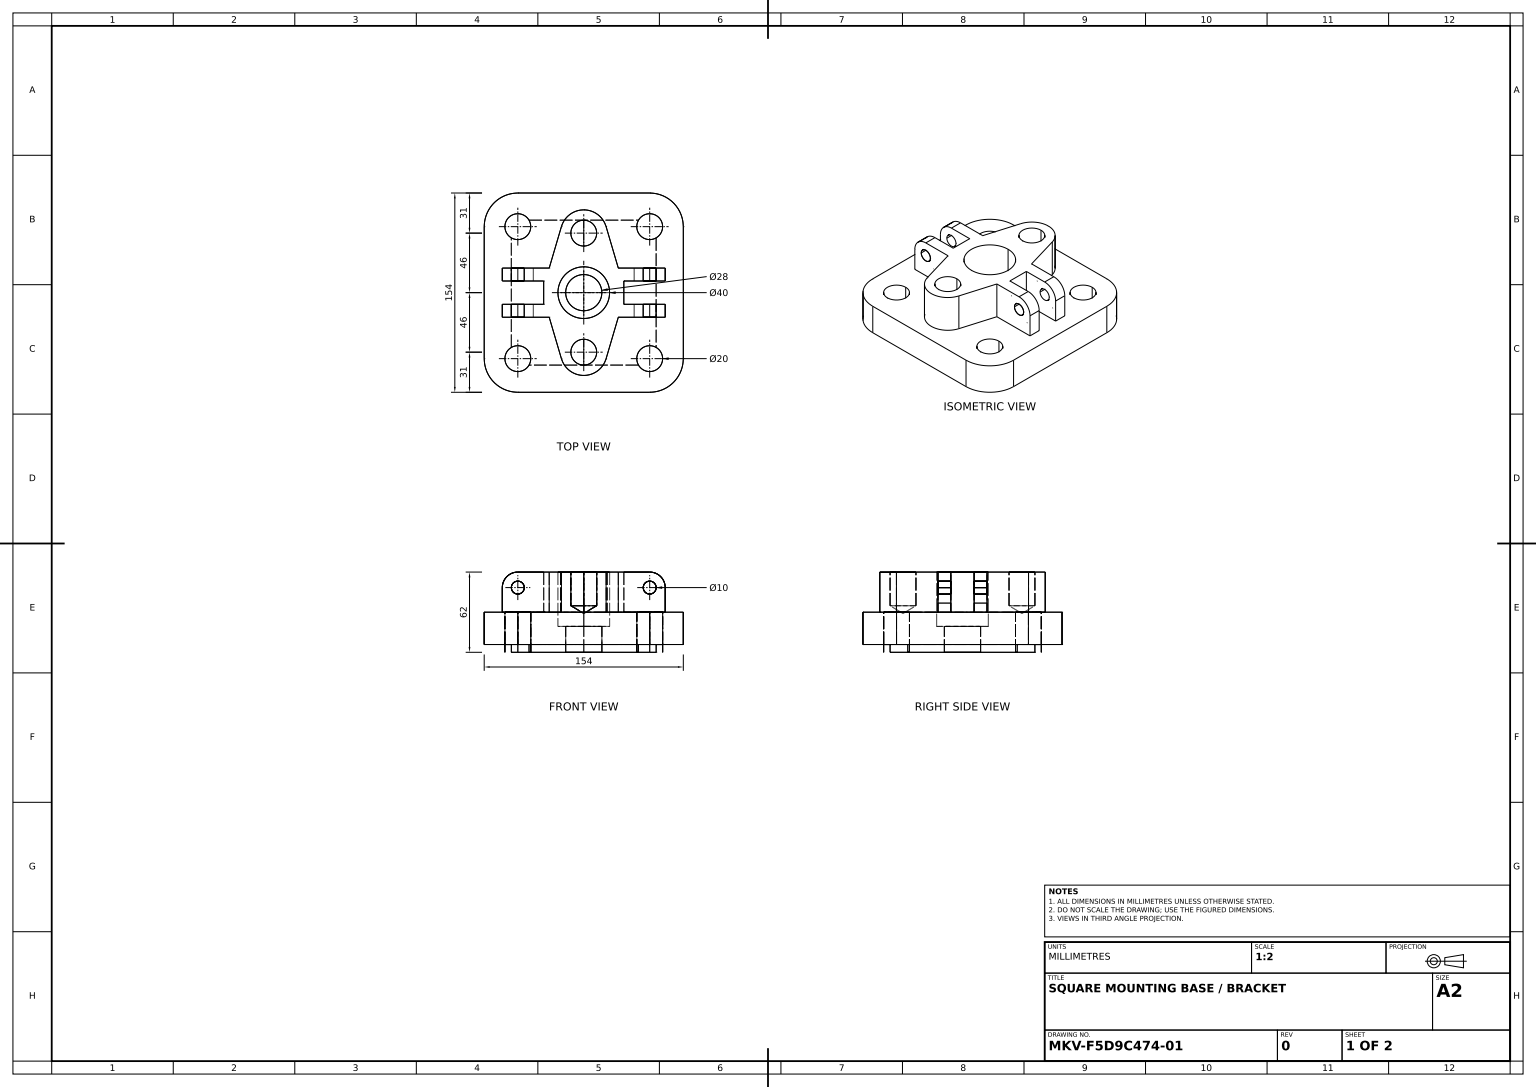
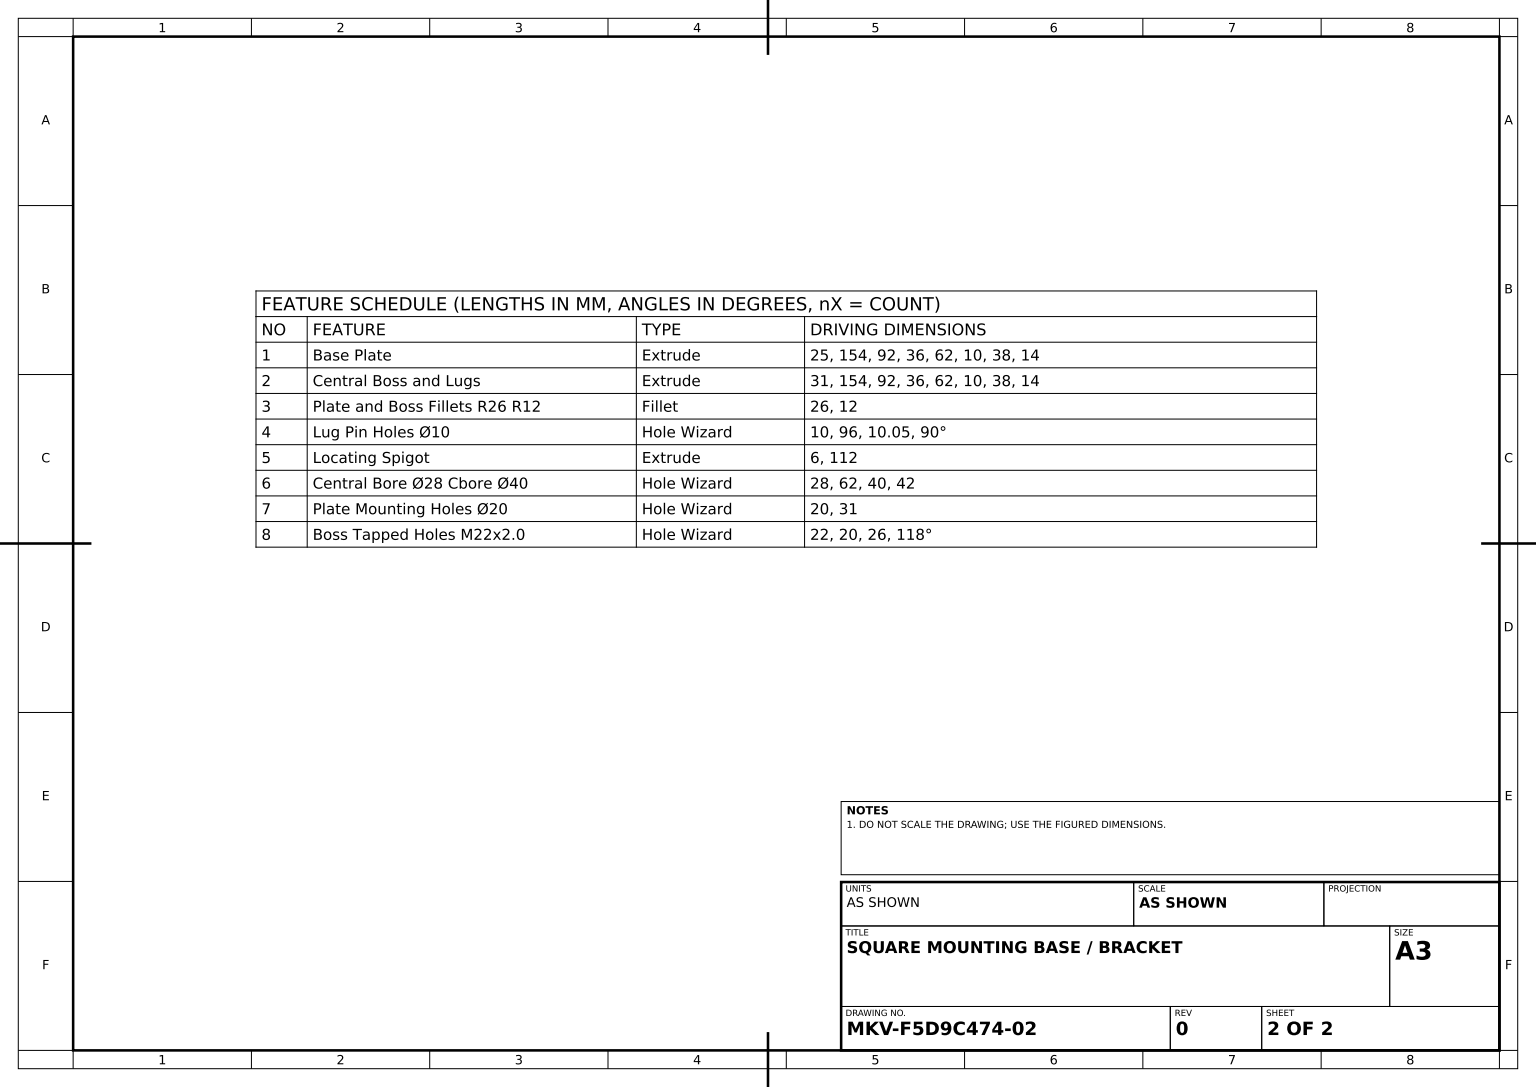
solid
v1 (0,14,-14)
v2 (0,14,14)
e1 v1 v2 CIRCLE(AX(P(0,14,0),D(0,1,0),D(0,0,1)),14)
v3 (0,-6,14)
e2 v3 v2 LINE
v4 (0,-6,-14)
e3 v4 v3 CIRCLE(AX(P(0,-6,0),D(0,1,0),D(0,0,1)),14)
e4 v4 v1 LINE
face CYL(AX(P(0,56,0),D(0,1,0),D(0,0,1)),14) rev [e1 -e2 -e3 e4]
v5 (31,56,-9)
v6 (51,56,-9)
e5 v5 v6 LINE
v7 (31,25,-9)
e6 v5 v7 LINE
v8 (63,25,-9)
e7 v7 v8 LINE
v9 (63,44,-9)
e8 v9 v8 LINE
e9 v9 v6 CIRCLE(AX(P(51,44,-9),D(0,0,1),D(-1,0,0)),12)
v10 (46,44,-9)
v11 (56,44,-9)
e10 v10 v11 CIRCLE(AX(P(51,44,-9),D(0,0,-1),D(-1,0,0)),5)
e11 v11 v10 CIRCLE(AX(P(51,44,-9),D(0,0,-1),D(-1,0,0)),5)
face PLANE(AX(P(0,56,-9),D(0,0,-1),D(-1,0,0))) rev [-e5 e6 e7 -e8 e9] [e10 e11]
v12 (-51,0,-77)
v13 (51,0,-77)
e12 v12 v13 LINE
v14 (-51,25,-77)
e13 v12 v14 LINE
v15 (51,25,-77)
e14 v14 v15 LINE
e15 v15 v13 LINE
face PLANE(AX(P(0,25,-77),D(0,0,-1),D(-1,0,0))) [-e12 e13 e14 e15]
v16 (0,30,-56)
v17 (0,30,-36)
e16 v16 v17 CIRCLE(AX(P(0,30,-46),D(0,1,0),D(0,0,1)),10)
v18 (0,23.991394,-46)
e17 v18 v17 LINE
e18 v18 v16 LINE
face CONE(AX(P(0,30,-46),D(0,1,0),D(0,0,1)),10,1.029744259) rev [e16 -e17 e18]
v19 (-31,25,9)
v20 (-63,25,9)
e19 v19 v20 LINE
v21 (-63,44,9)
e20 v21 v20 LINE
v22 (-51,56,9)
e21 v21 v22 CIRCLE(AX(P(-51,44,9),D(0,0,-1),D(1,0,0)),12)
v23 (-31,56,9)
e22 v23 v22 LINE
e23 v23 v19 LINE
v24 (-46,44,9)
v25 (-56,44,9)
e24 v24 v25 CIRCLE(AX(P(-51,44,9),D(0,0,1),D(1,0,0)),5)
e25 v25 v24 CIRCLE(AX(P(-51,44,9),D(0,0,1),D(1,0,0)),5)
face PLANE(AX(P(0,56,9),D(0,0,1),D(1,0,0))) rev [e19 -e20 e21 -e22 e23] [e24 e25]
v26 (56,44,18.975)
v27 (46,44,18.975)
e26 v26 v27 CIRCLE(AX(P(51,44,18.975),D(0,0,1),D(1,0,0)),5)
v28 (56.025,44,19)
e27 v26 v28 LINE
v29 (45.975,44,19)
e28 v28 v29 CIRCLE(AX(P(51,44,19),D(0,0,1),D(1,0,0)),5.025)
e29 v27 v29 LINE
face CONE(AX(P(51,44,19),D(0,0,1),D(1,0,0)),5.025,0.785398163) rev [-e26 e27 e28 -e29]
v30 (0,30,56)
v31 (0,30,36)
e30 v30 v31 CIRCLE(AX(P(0,30,46),D(0,1,0),D(0,0,1)),10)
v32 (0,23.991394,46)
e31 v32 v31 LINE
e32 v32 v30 LINE
face CONE(AX(P(0,30,46),D(0,1,0),D(0,0,1)),10,1.029744259) rev [e30 -e31 e32]
v33 (-26.719654,25,-19)
v34 (-17.266235,25,-51.086957)
e33 v33 v34 LINE
v35 (-26.719654,56,-19)
e34 v35 v33 LINE
v36 (-17.266235,56,-51.086957)
e35 v35 v36 LINE
e36 v36 v34 LINE
face PLANE(AX(P(-29.736294,56,-8.76087),D(-0.959235281,0,-0.282608696),D(-0.282608696,0,0.959235281))) [-e33 -e34 e35 e36]
v37 (51,0,77)
v38 (51,25,77)
e37 v37 v38 LINE
v39 (-51,25,77)
e38 v39 v38 LINE
v40 (-51,0,77)
e39 v39 v40 LINE
e40 v40 v37 LINE
face PLANE(AX(P(0,25,77),D(0,0,-1),D(-1,0,0))) rev [e37 -e38 e39 e40]
v41 (-42.339746,-6,-56)
v42 (-42.339746,0,-56)
e41 v41 v42 LINE
v43 (42.339746,0,-56)
e42 v42 v43 LINE
v44 (42.339746,-6,-56)
e43 v43 v44 LINE
e44 v41 v44 LINE
face PLANE(AX(P(-56,-6,-56),D(0,0,1),D(1,0,0))) rev [e41 e42 e43 -e44]
v45 (51,0,-61)
v46 (51,25,-61)
e45 v45 v46 LINE
v47 (51,25,-41)
e46 v46 v47 CIRCLE(AX(P(51,25,-51),D(0,1,0),D(0,0,1)),10)
v48 (51,-6,-41)
e47 v48 v47 LINE
e48 v44 v48 CIRCLE(AX(P(51,-6,-51),D(0,1,0),D(0,0,1)),10)
e49 v45 v43 CIRCLE(AX(P(51,0,-51),D(0,1,0),D(0,0,1)),10)
face CYL(AX(P(51,25,-51),D(0,1,0),D(0,0,1)),10) rev [e45 e46 -e47 -e48 -e43 -e49]
v49 (0,56,-36)
v50 (0,56,-56)
e50 v49 v50 CIRCLE(AX(P(0,56,-46),D(0,1,0),D(0,0,1)),10)
e51 v16 v50 LINE
e52 v17 v16 CIRCLE(AX(P(0,30,-46),D(0,1,0),D(0,0,1)),10)
e53 v17 v49 LINE
face CYL(AX(P(0,56,-46),D(0,1,0),D(0,0,1)),10) rev [e50 -e51 -e52 e53]
v51 (-77,25,51)
e54 v51 v39 CIRCLE(AX(P(-51,25,51),D(0,1,0),D(0,0,1)),26)
v52 (-77,0,51)
e55 v52 v51 LINE
e56 v40 v52 CIRCLE(AX(P(-51,0,51),D(0,-1,0),D(0,0,1)),26)
face CYL(AX(P(-51,25,51),D(0,-1,0),D(0,0,-1)),26) [-e39 -e54 -e55 -e56]
e57 v50 v49 CIRCLE(AX(P(0,56,-46),D(0,1,0),D(0,0,1)),10)
face CYL(AX(P(0,56,-46),D(0,1,0),D(0,0,1)),10) rev [e57 -e53 -e16 e51]
v53 (-51,-6,-41)
v54 (-51,25,-41)
e58 v53 v54 LINE
v55 (-56,-6,-42.339746)
e59 v55 v53 CIRCLE(AX(P(-51,-6,-51),D(0,1,0),D(0,0,1)),10)
v56 (-56,0,-42.339746)
e60 v56 v55 LINE
v57 (-51,0,-61)
e61 v57 v56 CIRCLE(AX(P(-51,0,-51),D(0,1,0),D(0,0,1)),10)
v58 (-51,25,-61)
e62 v57 v58 LINE
e63 v58 v54 CIRCLE(AX(P(-51,25,-51),D(0,1,0),D(0,0,1)),10)
face CYL(AX(P(-51,25,-51),D(0,1,0),D(0,0,1)),10) rev [-e58 -e59 -e60 -e61 e62 e63]
v59 (51,56,19)
v60 (51,56,9)
e64 v59 v60 LINE
v61 (63,44,19)
e65 v61 v59 CIRCLE(AX(P(51,44,19),D(0,0,1),D(-1,0,0)),12)
v62 (63,44,9)
e66 v62 v61 LINE
e67 v60 v62 CIRCLE(AX(P(51,44,9),D(0,0,-1),D(-1,0,0)),12)
face CYL(AX(P(51,44,0),D(0,0,1),D(1,0,0)),12) [-e64 -e65 -e66 -e67]
v63 (26.719654,56,-19)
v64 (51,56,-19)
e68 v63 v64 LINE
v65 (63,44,-19)
e69 v64 v65 CIRCLE(AX(P(51,44,-19),D(0,0,-1),D(-1,0,0)),12)
v66 (63,25,-19)
e70 v65 v66 LINE
v67 (26.719654,25,-19)
e71 v67 v66 LINE
e72 v63 v67 LINE
v68 (46,44,-19)
v69 (56,44,-19)
e73 v68 v69 CIRCLE(AX(P(51,44,-19),D(0,0,-1),D(-1,0,0)),5)
e74 v69 v68 CIRCLE(AX(P(51,44,-19),D(0,0,-1),D(-1,0,0)),5)
face PLANE(AX(P(0,56,-19),D(0,0,-1),D(-1,0,0))) [e68 e69 e70 -e71 -e72] [-e73 -e74]
e75 v69 v11 LINE
e76 v68 v10 LINE
face CYL(AX(P(51,44,19),D(0,0,1),D(1,0,0)),5) rev [-e11 -e75 e74 e76]
e77 v42 v57 CIRCLE(AX(P(-51,0,-51),D(0,1,0),D(0,0,1)),10)
v70 (-56,0,42.339746)
e78 v70 v56 LINE
v71 (-51,0,61)
e79 v70 v71 CIRCLE(AX(P(-51,0,51),D(0,1,0),D(0,0,1)),10)
v72 (-42.339746,0,56)
e80 v71 v72 CIRCLE(AX(P(-51,0,51),D(0,1,0),D(0,0,1)),10)
v73 (42.339746,0,56)
e81 v73 v72 LINE
v74 (51,0,61)
e82 v73 v74 CIRCLE(AX(P(51,0,51),D(0,1,0),D(0,0,1)),10)
v75 (56,0,42.339746)
e83 v74 v75 CIRCLE(AX(P(51,0,51),D(0,1,0),D(0,0,1)),10)
v76 (56,0,-42.339746)
e84 v76 v75 LINE
e85 v76 v45 CIRCLE(AX(P(51,0,-51),D(0,1,0),D(0,0,1)),10)
v77 (77,0,-51)
e86 v13 v77 CIRCLE(AX(P(51,0,-51),D(0,-1,0),D(0,0,1)),26)
v78 (77,0,51)
e87 v77 v78 LINE
e88 v78 v37 CIRCLE(AX(P(51,0,51),D(0,-1,0),D(0,0,1)),26)
v79 (-77,0,-51)
e89 v79 v52 LINE
e90 v79 v12 CIRCLE(AX(P(-51,0,-51),D(0,-1,0),D(0,0,1)),26)
face PLANE(AX(P(0,0,0),D(0,1,0),D(0,0,1))) rev [e77 e61 -e78 e79 e80 -e81 e82 e83 -e84 e85 e49 -e42] [e12 e86 e87 e88 -e40 e56 -e89 e90]
v80 (56,44,9)
v81 (46,44,9)
e91 v80 v81 CIRCLE(AX(P(51,44,9),D(0,0,-1),D(-1,0,0)),5)
e92 v81 v80 CIRCLE(AX(P(51,44,9),D(0,0,-1),D(-1,0,0)),5)
v82 (31,56,9)
e93 v82 v60 LINE
v83 (63,25,9)
e94 v62 v83 LINE
v84 (31,25,9)
e95 v84 v83 LINE
e96 v82 v84 LINE
face PLANE(AX(P(0,56,9),D(0,0,-1),D(-1,0,0))) [-e91 -e92] [e93 e67 e94 -e95 -e96]
e97 v27 v26 CIRCLE(AX(P(51,44,18.975),D(0,0,1),D(1,0,0)),5)
e98 v29 v28 CIRCLE(AX(P(51,44,19),D(0,0,1),D(1,0,0)),5.025)
face CONE(AX(P(51,44,19),D(0,0,1),D(1,0,0)),5.025,0.785398163) rev [-e97 e29 e98 -e27]
v85 (-46,44,-19)
v86 (-56,44,-19)
e99 v85 v86 CIRCLE(AX(P(-51,44,-19),D(0,0,1),D(1,0,0)),5)
v87 (-46,44,-9)
e100 v85 v87 LINE
v88 (-56,44,-9)
e101 v87 v88 CIRCLE(AX(P(-51,44,-9),D(0,0,1),D(1,0,0)),5)
e102 v86 v88 LINE
face CYL(AX(P(-51,44,19),D(0,0,1),D(1,0,0)),5) rev [-e99 e100 e101 -e102]
face CONE(AX(P(0,30,-46),D(0,1,0),D(0,0,1)),10,1.029744259) rev [e17 e52 -e18]
v89 (0,56,56)
e103 v30 v89 LINE
e104 v31 v30 CIRCLE(AX(P(0,30,46),D(0,1,0),D(0,0,1)),10)
v90 (0,56,36)
e105 v31 v90 LINE
e106 v90 v89 CIRCLE(AX(P(0,56,46),D(0,1,0),D(0,0,1)),10)
face CYL(AX(P(0,56,46),D(0,1,0),D(0,0,1)),10) rev [-e103 -e104 e105 e106]
v91 (77,25,-51)
v92 (77,25,51)
e107 v91 v92 LINE
e108 v92 v78 LINE
e109 v77 v91 LINE
face PLANE(AX(P(77,25,0),D(1,0,0),D(0,0,-1))) [e107 e108 -e87 e109]
v93 (-26.719654,25,19)
v94 (-17.266235,25,51.086957)
e110 v93 v94 LINE
v95 (-17.266235,56,51.086957)
e111 v95 v94 LINE
v96 (-26.719654,56,19)
e112 v96 v95 LINE
e113 v96 v93 LINE
face PLANE(AX(P(-29.736294,56,8.76087),D(0.959235281,0,-0.282608696),D(-0.282608696,0,-0.959235281))) rev [e110 -e111 -e112 e113]
v97 (56,-6,-42.339746)
e114 v97 v76 LINE
e115 v48 v97 CIRCLE(AX(P(51,-6,-51),D(0,1,0),D(0,0,1)),10)
e116 v47 v46 CIRCLE(AX(P(51,25,-51),D(0,1,0),D(0,0,1)),10)
face CYL(AX(P(51,25,-51),D(0,1,0),D(0,0,1)),10) rev [-e85 -e114 -e115 e47 e116 -e45]
v98 (-31,56,-9)
v99 (-31,25,-9)
e117 v98 v99 LINE
e118 v19 v99 LINE
e119 v23 v98 LINE
face PLANE(AX(P(-31,56,0),D(-1,0,0),D(0,0,1))) [e117 -e118 -e23 e119]
e120 v53 v41 CIRCLE(AX(P(-51,-6,-51),D(0,1,0),D(0,0,1)),10)
e121 v54 v58 CIRCLE(AX(P(-51,25,-51),D(0,1,0),D(0,0,1)),10)
face CYL(AX(P(-51,25,-51),D(0,1,0),D(0,0,1)),10) rev [-e41 -e120 e58 e121 -e62 -e77]
v100 (-46,44,18.975)
v101 (-56,44,18.975)
e122 v100 v101 CIRCLE(AX(P(-51,44,18.975),D(0,0,1),D(1,0,0)),5)
v102 (-45.975,44,19)
e123 v100 v102 LINE
v103 (-56.025,44,19)
e124 v102 v103 CIRCLE(AX(P(-51,44,19),D(0,0,1),D(1,0,0)),5.025)
e125 v101 v103 LINE
face CONE(AX(P(-51,44,19),D(0,0,1),D(1,0,0)),5.025,0.785398163) rev [-e122 e123 e124 -e125]
e126 v88 v87 CIRCLE(AX(P(-51,44,-9),D(0,0,1),D(1,0,0)),5)
v104 (-51,56,-9)
e127 v98 v104 LINE
v105 (-63,44,-9)
e128 v104 v105 CIRCLE(AX(P(-51,44,-9),D(0,0,1),D(1,0,0)),12)
v106 (-63,25,-9)
e129 v105 v106 LINE
e130 v99 v106 LINE
face PLANE(AX(P(0,56,-9),D(0,0,1),D(1,0,0))) [-e126 -e101] [-e117 e127 e128 e129 -e130]
e131 v103 v102 CIRCLE(AX(P(-51,44,19),D(0,0,1),D(1,0,0)),5.025)
e132 v101 v100 CIRCLE(AX(P(-51,44,18.975),D(0,0,1),D(1,0,0)),5)
face CONE(AX(P(-51,44,19),D(0,0,1),D(1,0,0)),5.025,0.785398163) rev [e125 e131 -e123 -e132]
v107 (-63,44,-19)
e133 v105 v107 LINE
v108 (-51,56,-19)
e134 v108 v104 LINE
e135 v107 v108 CIRCLE(AX(P(-51,44,-19),D(0,0,-1),D(1,0,0)),12)
face CYL(AX(P(-51,44,0),D(0,0,-1),D(-1,0,0)),12) [-e133 -e128 -e134 -e135]
v109 (56,-6,42.339746)
v110 (51,-6,41)
e136 v109 v110 CIRCLE(AX(P(51,-6,51),D(0,1,0),D(0,0,1)),10)
e137 v75 v109 LINE
v111 (51,25,61)
e138 v74 v111 LINE
v112 (51,25,41)
e139 v111 v112 CIRCLE(AX(P(51,25,51),D(0,1,0),D(0,0,1)),10)
e140 v110 v112 LINE
face CYL(AX(P(51,25,51),D(0,1,0),D(0,0,1)),10) rev [-e136 -e137 -e83 e138 e139 -e140]
e141 v6 v64 LINE
e142 v65 v9 LINE
face CYL(AX(P(51,44,-46),D(0,0,1),D(1,0,0)),12) [-e141 -e9 -e142 -e69]
v113 (42.339746,-6,56)
e143 v113 v73 LINE
e144 v110 v113 CIRCLE(AX(P(51,-6,51),D(0,1,0),D(0,0,1)),10)
e145 v112 v111 CIRCLE(AX(P(51,25,51),D(0,1,0),D(0,0,1)),10)
face CYL(AX(P(51,25,51),D(0,1,0),D(0,0,1)),10) rev [-e138 -e82 -e143 -e144 e140 e145]
v114 (17.266235,25,51.086957)
e146 v94 v114 CIRCLE(AX(P(0,25,46),D(0,1,0),D(0,0,1)),18)
v115 (17.266235,56,51.086957)
e147 v115 v114 LINE
e148 v95 v115 CIRCLE(AX(P(0,56,46),D(0,1,0),D(0,0,1)),18)
face CYL(AX(P(0,56,46),D(0,-1,0),D(0,0,-1)),18) [e146 -e147 -e148 e111]
v116 (-77,25,-51)
e149 v116 v79 LINE
e150 v14 v116 CIRCLE(AX(P(-51,25,-51),D(0,1,0),D(0,0,1)),26)
face CYL(AX(P(-51,25,-51),D(0,1,0),D(0,0,1)),26) [-e13 -e90 -e149 -e150]
v117 (0,14,-20)
v118 (0,56,-20)
e151 v117 v118 LINE
v119 (0,56,20)
e152 v118 v119 CIRCLE(AX(P(0,56,0),D(0,1,0),D(0,0,1)),20)
v120 (0,14,20)
e153 v120 v119 LINE
e154 v117 v120 CIRCLE(AX(P(0,14,0),D(0,1,0),D(0,0,1)),20)
face CYL(AX(P(0,56,0),D(0,1,0),D(0,0,1)),20) rev [e151 e152 -e153 -e154]
v121 (-63,44,19)
v122 (-63,25,19)
e155 v121 v122 LINE
e156 v93 v122 LINE
v123 (-51,56,19)
e157 v96 v123 LINE
e158 v123 v121 CIRCLE(AX(P(-51,44,19),D(0,0,1),D(1,0,0)),12)
face PLANE(AX(P(0,56,19),D(0,0,1),D(1,0,0))) [-e131 -e124] [e155 -e156 -e113 e157 e158]
v124 (26.719654,56,19)
v125 (26.719654,25,19)
e159 v124 v125 LINE
v126 (63,25,19)
e160 v125 v126 LINE
e161 v61 v126 LINE
e162 v124 v59 LINE
face PLANE(AX(P(0,56,19),D(0,0,-1),D(-1,0,0))) rev [e159 e160 -e161 e65 -e162] [-e28 -e98]
e163 v116 v51 LINE
face PLANE(AX(P(-77,25,0),D(1,0,0),D(0,0,-1))) rev [-e163 e149 e89 e55]
v127 (-56,-6,42.339746)
e164 v127 v55 LINE
e165 v97 v109 LINE
v128 (-42.339746,-6,56)
e166 v113 v128 LINE
v129 (-51,-6,41)
e167 v128 v129 CIRCLE(AX(P(-51,-6,51),D(0,1,0),D(0,0,1)),10)
e168 v129 v127 CIRCLE(AX(P(-51,-6,51),D(0,1,0),D(0,0,1)),10)
e169 v3 v4 CIRCLE(AX(P(0,-6,0),D(0,1,0),D(0,0,1)),14)
face PLANE(AX(P(0,-6,0),D(0,-1,0),D(0,0,-1))) [e164 e59 e120 e44 e48 e115 e165 e136 e144 e166 e167 e168] [e3 e169]
e170 v119 v118 CIRCLE(AX(P(0,56,0),D(0,1,0),D(0,0,1)),20)
e171 v120 v117 CIRCLE(AX(P(0,14,0),D(0,1,0),D(0,0,1)),20)
face CYL(AX(P(0,56,0),D(0,1,0),D(0,0,1)),20) rev [e170 -e151 -e171 e153]
e172 v72 v128 LINE
face PLANE(AX(P(-56,-6,56),D(0,0,-1),D(-1,0,0))) rev [e172 -e166 e143 e81]
face CYL(AX(P(51,44,19),D(0,0,1),D(1,0,0)),5) rev [-e76 e73 e75 -e10]
e173 v89 v90 CIRCLE(AX(P(0,56,46),D(0,1,0),D(0,0,1)),10)
face CYL(AX(P(0,56,46),D(0,1,0),D(0,0,1)),10) rev [-e105 -e30 e103 e173]
e174 v91 v15 CIRCLE(AX(P(51,25,-51),D(0,1,0),D(0,0,1)),26)
face CYL(AX(P(51,25,-51),D(0,-1,0),D(0,0,-1)),26) [-e86 -e15 -e174 -e109]
e175 v124 v115 LINE
e176 v125 v114 LINE
face PLANE(AX(P(29.736294,56,8.76087),D(0.959235281,0,0.282608696),D(0.282608696,0,-0.959235281))) [e175 e147 -e176 -e159]
e177 v25 v101 LINE
e178 v24 v100 LINE
face CYL(AX(P(-51,44,19),D(0,0,1),D(1,0,0)),5) rev [-e177 -e24 e178 e122]
e179 v86 v85 CIRCLE(AX(P(-51,44,-19),D(0,0,1),D(1,0,0)),5)
v130 (-63,25,-19)
e180 v107 v130 LINE
e181 v35 v108 LINE
e182 v33 v130 LINE
face PLANE(AX(P(0,56,-19),D(0,0,1),D(1,0,0))) rev [e179 e99] [-e180 e135 -e181 e34 e182]
e183 v127 v70 LINE
face PLANE(AX(P(-56,-6,56),D(1,0,0),D(0,0,-1))) rev [e78 e60 -e164 e183]
e184 v20 v122 LINE
e185 v121 v21 LINE
face PLANE(AX(P(-63,56,0),D(1,0,0),D(0,0,-1))) rev [e184 -e155 e185 e20]
e186 v22 v123 LINE
e187 v82 v5 LINE
v131 (17.266235,56,-51.086957)
e188 v63 v131 LINE
v132 (0,56,-64)
e189 v131 v132 CIRCLE(AX(P(0,56,-46),D(0,1,0),D(0,0,1)),18)
e190 v132 v36 CIRCLE(AX(P(0,56,-46),D(0,1,0),D(0,0,1)),18)
face PLANE(AX(P(0,56,-46),D(0,1,0),D(0,0,1))) [-e173 -e106] [-e50 -e57] [-e127 -e119 e22 e186 -e157 e112 e148 -e175 e162 e64 -e93 e187 e5 e141 -e68 e188 e189 e190 -e35 e181 e134] [-e152 -e170]
v133 (0,25,-64)
e191 v132 v133 LINE
e192 v133 v34 CIRCLE(AX(P(0,25,-46),D(0,1,0),D(0,0,1)),18)
face CYL(AX(P(0,56,-46),D(0,-1,0),D(0,0,-1)),18) [-e190 e191 e192 -e36]
face CONE(AX(P(0,30,46),D(0,1,0),D(0,0,1)),10,1.029744259) rev [-e32 e31 e104]
face CYL(AX(P(-51,44,19),D(0,0,1),D(1,0,0)),5) rev [-e25 e177 e132 -e178]
v134 (17.266235,25,-51.086957)
e193 v131 v134 LINE
e194 v67 v134 LINE
face PLANE(AX(P(29.736294,56,-8.76087),D(-0.959235281,0,0.282608696),D(0.282608696,0,0.959235281))) rev [-e193 -e188 e72 e194]
e195 v2 v1 CIRCLE(AX(P(0,14,0),D(0,1,0),D(0,0,1)),14)
face CYL(AX(P(0,56,0),D(0,1,0),D(0,0,1)),14) rev [e2 e195 -e4 -e169]
face PLANE(AX(P(14,14,0),D(0,-1,0),D(0,0,-1))) rev [e171 e154] [-e1 -e195]
face CYL(AX(P(-51,44,19),D(0,0,1),D(1,0,0)),5) rev [-e100 -e179 e102 e126]
e196 v83 v126 LINE
face PLANE(AX(P(63,56,0),D(1,0,0),D(0,0,-1))) [-e196 -e94 e66 e161]
e197 v106 v130 LINE
face PLANE(AX(P(-63,56,0),D(-1,0,0),D(0,0,1))) [-e129 e133 e180 -e197]
v135 (-51,25,41)
v136 (-51,25,61)
e198 v135 v136 CIRCLE(AX(P(-51,25,51),D(0,1,0),D(0,0,1)),10)
e199 v136 v135 CIRCLE(AX(P(-51,25,51),D(0,1,0),D(0,0,1)),10)
e200 v38 v92 CIRCLE(AX(P(51,25,51),D(0,1,0),D(0,0,1)),26)
e201 v8 v66 LINE
e202 v84 v7 LINE
e203 v134 v133 CIRCLE(AX(P(0,25,-46),D(0,1,0),D(0,0,1)),18)
face PLANE(AX(P(0,25,0),D(0,1,0),D(0,0,1))) [-e198 -e199] [e38 e200 -e107 e174 -e14 e150 e163 e54] [-e201 -e7 -e202 e95 e196 -e160 e176 -e146 -e110 e156 -e184 -e19 e118 e130 e197 -e182 e33 -e192 -e203 -e194 e71] [-e145 -e139] [-e121 -e63] [-e116 -e46]
face PLANE(AX(P(31,56,0),D(-1,0,0),D(0,0,1))) rev [-e6 -e187 e96 e202]
e204 v71 v136 LINE
e205 v129 v135 LINE
face CYL(AX(P(-51,25,51),D(0,1,0),D(0,0,1)),10) rev [-e172 -e80 e204 e199 -e205 -e167]
face CYL(AX(P(-51,25,51),D(0,1,0),D(0,0,1)),10) rev [-e79 -e183 -e168 e205 e198 -e204]
e206 v81 v27 LINE
e207 v80 v26 LINE
face CYL(AX(P(51,44,19),D(0,0,1),D(1,0,0)),5) rev [e91 e206 e97 -e207]
face CYL(AX(P(51,44,19),D(0,0,1),D(1,0,0)),5) rev [-e206 e92 e207 e26]
face CYL(AX(P(0,56,-46),D(0,-1,0),D(0,0,-1)),18) [-e191 -e189 e193 e203]
face CYL(AX(P(51,25,51),D(0,1,0),D(0,0,1)),26) [-e200 -e37 -e88 -e108]
face PLANE(AX(P(63,56,0),D(-1,0,0),D(0,0,1))) rev [-e70 e142 e8 e201]
face CYL(AX(P(-51,44,-46),D(0,0,-1),D(-1,0,0)),12) [-e158 -e186 -e21 -e185]
face PLANE(AX(P(56,-6,56),D(-1,0,0),D(0,0,1))) rev [e137 -e165 e114 e84]
